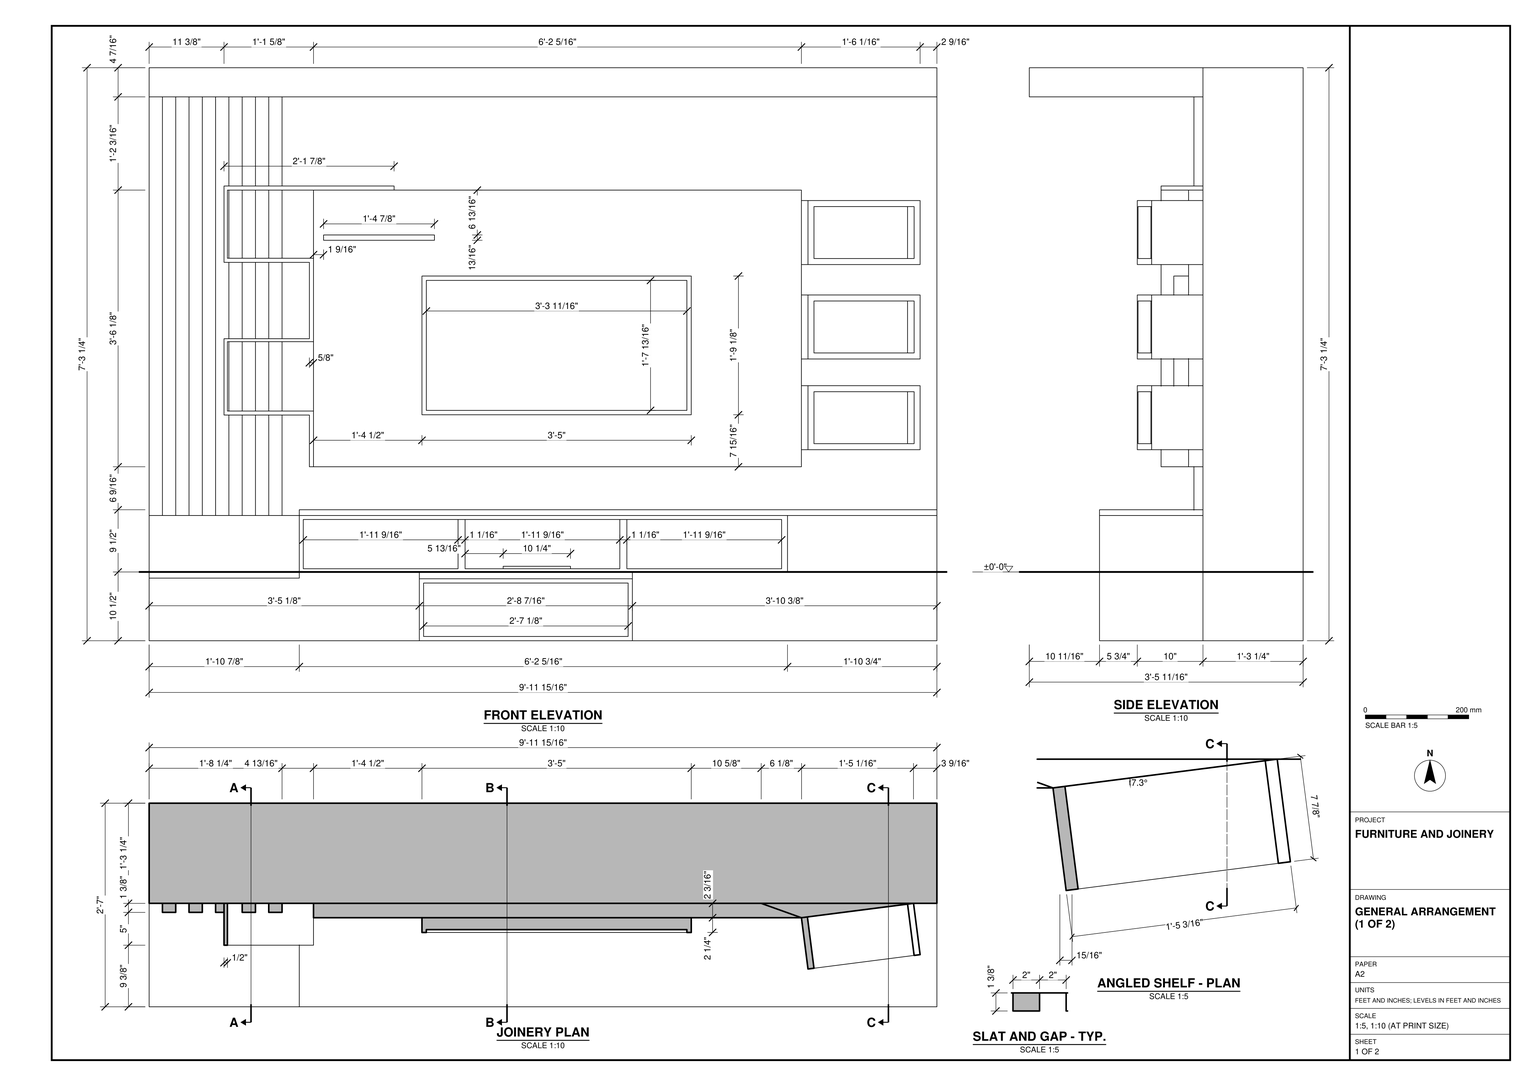
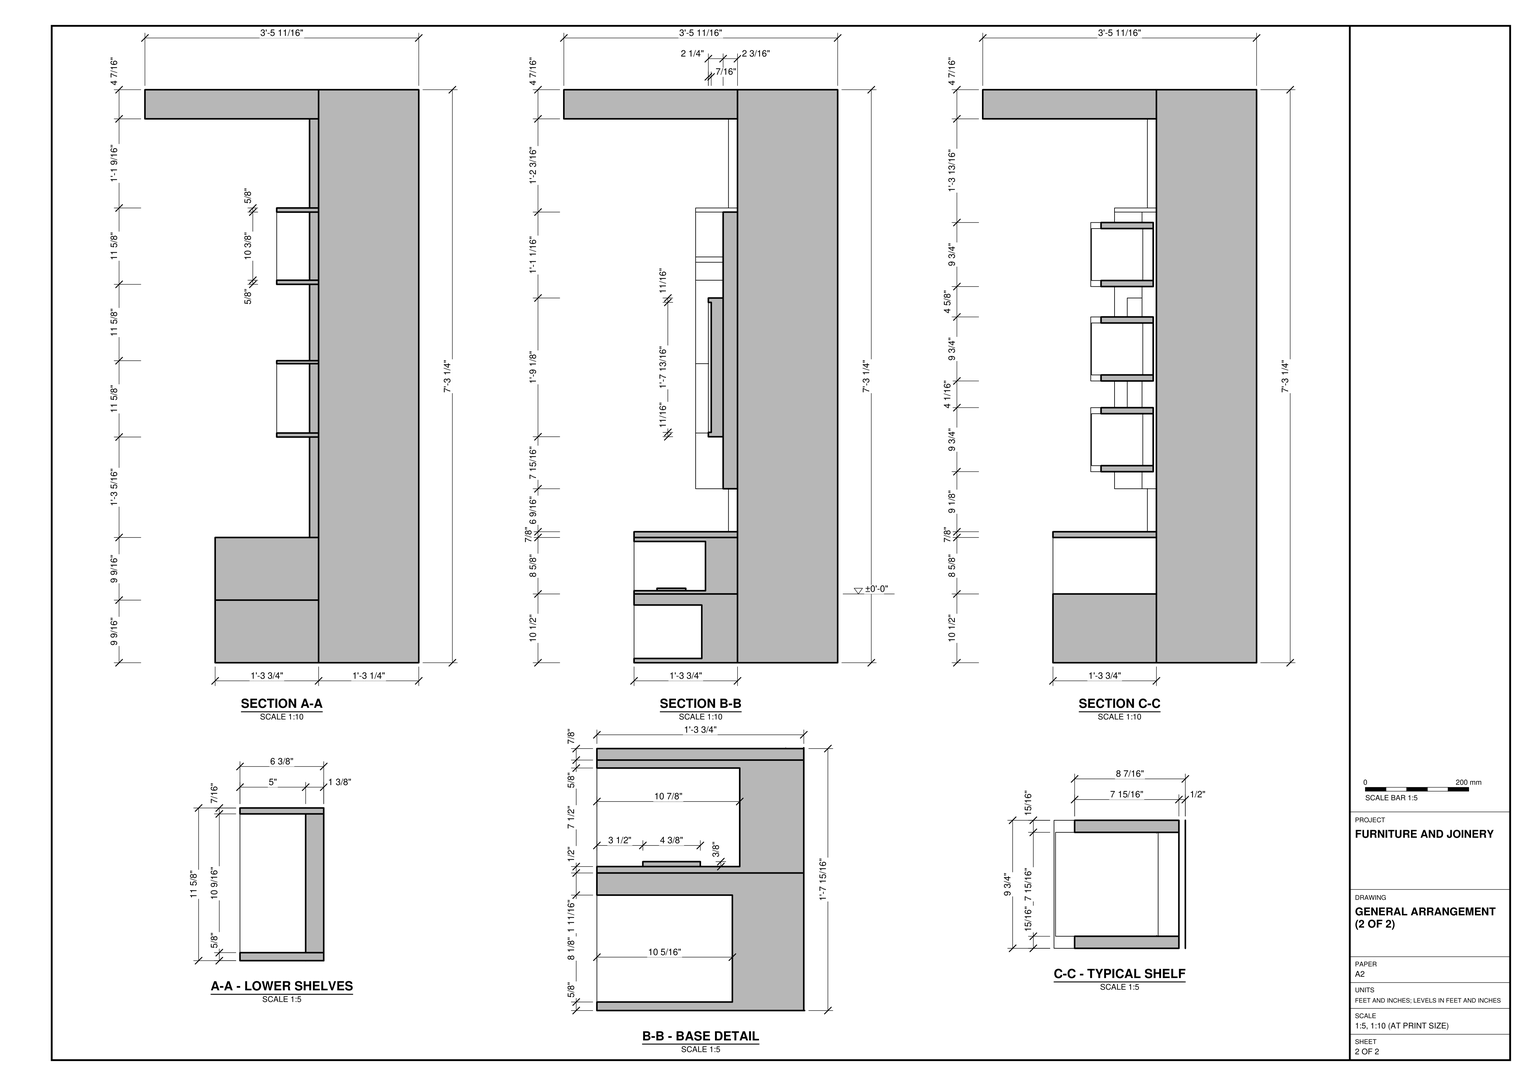
Build the media wall in SketchUp using task_files/diagram_01.pdf. Work in feet and inches. The complete unit is 9'-11 15/16" wide, 3'-5 11/16" deep and 7'-3 1/4" high. Use the ±0'-0" datum shown at the division between the two base tiers; the bottom of the unit is 10 1/2" below it.

Use the front elevation to lay out the full-height backing, the projecting top canopy and the low storage base. On the left, run the vertical slats from the base to the canopy and fit the open shelf returns in front of them. Set the broad rectangular panel forward of the backing. Include the framed display on its face and the short shelf above and to the left of the display. Stack the open box shelves at the right edge of the panel, using the angled shelf plan to orient them. In the base, form the row of three upper compartments and the wider single opening below.

Use sections A-A, B-B and C-C and their details to set board thicknesses, recess depths and projections so the joinery matches in side view as well as in elevation. Keep the backing, canopy, panel, shelving and base storage as separate groups or components, and use components for repeated parts. Any decor or loose items may be suitable library components, for example from 3D Warehouse. Save one SketchUp model as output_files/media_wall_with_display_shelving_and_base_storage.skp.

# SketchUp Ruby script. Lengths in inches.
U = 1.inch
M = Sketchup.active_model
def pt(a) = Geom::Point3d.new(a.map { |v| v * U })
def face(e, loops, mat)
  f = e.add_face(loops[0].map { |a| pt(a) })
  loops[1..].each { |l| e.add_face(l.map { |a| pt(a) }).erase! }
  f.material = f.back_material = mat if mat
  f
end
# faces: each face lists its corners as indices into pts; further lists are holes
def faces(e, pts, list, mat = nil) = list.each { |f| face(e, (f[0].is_a?(Array) ? f : [f]).map { |l| l.map { |i| pts[i] } }, mat) }
# xy, xz, yz: faces in a plane at the given z, y or x. An outline is a flat list of corners, or four numbers for a rectangle; further outlines are holes
def ring(l) = l.size == 4 ? [[l[0], l[1]], [l[2], l[1]], [l[2], l[3]], [l[0], l[3]]] : l.each_slice(2).to_a
def flat(e, list, mat, &to3) = list.each { |f| face(e, (f[0].is_a?(Array) ? f : [f]).map { |l| ring(l).map { |u, v| to3.(u, v) } }, mat) }
def xy(e, z, list, mat = nil) = flat(e, list, mat) { |x, y| [x, y, z] }
def xz(e, y, list, mat = nil) = flat(e, list, mat) { |x, z| [x, y, z] }
def yz(e, x, list, mat = nil) = flat(e, list, mat) { |y, z| [x, y, z] }
def lines(e, pts, list) = list.each { |a, b| e.add_line(pt(pts[a]), pt(pts[b])) }
# prism: a flat outline (further loops are holes) pulled along v
def prism(e, loops, v, mat = nil)
  f = face(e, loops, mat); d = Geom::Vector3d.new(v.map { |x| x * U })
  f.pushpull(f.normal.samedirection?(d) ? d.length : -d.length)
end
def box(e, o, s, mat = nil) = prism(e, [[o, [o[0] + s[0], o[1], o[2]], [o[0] + s[0], o[1] + s[1], o[2]], [o[0], o[1] + s[1], o[2]]]], [0, 0, s[2]], mat)
def at(x, y, z, deg = 0) = Geom::Transformation.translation(pt([x, y, z])) * Geom::Transformation.rotation(ORIGIN, Z_AXIS, deg.degrees)
def axes(o, x, y, z) = Geom::Transformation.new([*x, 0, *y, 0, *z, 0, *pt(o).to_a, 1])
def part(name) = M.definitions.add(name)
# library, detail: a bought-in or finely detailed component or shape, given as its bounding box
def library(name, o, s) = part(name).tap { |d| box(d.entities, o, s) }
def detail(e, o, s) = box(e.add_group.entities, o, s)
def put(e, d, t, mat = nil) = e.add_instance(d, t).tap { |i| i.material = mat if mat }
def group(e, t, mat = nil) = e.add_group.tap { |g| g.transformation = t; g.material = mat if mat }.entities
root = M.entities
M.materials.add("[0010_Snow]").color = [255, 250, 250]
M.materials.add("[Color M09]").color = [0, 0, 0]
M.materials.add("[Wood Bamboo]").color = [193, 114, 47]
M.materials.add("[Wood Bamboo]1").color = [177, 105, 43]
M.materials.add("[Wood Cherry Original]").color = [163, 92, 45]
M.materials.add("[Wood Cherry Original]1").color = [152, 86, 42]
xy(root,19.875,[[0,10.6875,119.9375,26.4375],[0,26.4375,119.9375,41.6875]])
xy(root,20.52,[[41.79,10.6875,72.92,21]],"[Wood Bamboo]")
xy(root,28.66,[[41.79,10.6875,72.92,21]],"[Wood Bamboo]")
xy(root,29.41,[[0,10.6875,22.86,26.4375]])
xy(root,30.35,[[22.86,10.6875,97.19,26.4375],[97.19,10.6875,119.9375,26.4375]])
xy(root,30.84,[[23.47,10.6875,47.03,21.5625],[[48.1,10.6875,71.66,21.5625],[53.9,14.19,64.15,18.56]],[72.73,10.6875,96.3,21.5625],[53.9,14.19,64.15,18.56]])
xy(root,31.21,[[53.9,14.19,64.15,18.56]],"[Color M09]")
xy(root,38.34,[[23.47,10.6875,47.03,21.5625],[48.1,10.6875,71.66,21.5625],[72.73,10.6875,96.3,21.5625]])
xy(root,38.94,[[0,10.6875,22.86,10.6875,22.86,26.4375,20.23,26.4375,20.23,25.0625,18.21,25.0625,18.21,26.4375,16.1875,26.4375,16.1875,25.0625,14.16,25.0625,14.16,26.4375,12.14,26.4375,12.14,25.0625,10.12,25.0625,10.12,26.4375,8.09,26.4375,8.09,25.0625,6.07,25.0625,6.07,26.4375,4.05,26.4375,4.05,25.0625,2.02,25.0625,2.02,26.4375,0,26.4375],[22.86,10.6875,97.19,26.4375],[2.02,25.0625,4.05,26.4375],[6.07,25.0625,8.09,26.4375],[10.12,25.0625,12.14,26.4375],
  [14.16,25.0625,16.1875,26.4375],[18.21,25.0625,20.23,26.4375]])
xy(root,38.94,[[97.19,10.6875,119.9375,26.4375]],"[Wood Bamboo]1")
xy(root,39.82,[[22.86,10.6875,119.9375,26.4375]],"[Wood Bamboo]1")
xy(root,46.36,[[24.4,20.0625,25.02,26.4375],[25.02,24.25,25.02,26.4375,93.18,26.4375,99.31,24.25]])
xy(root,48.96,[[100.31,16.4375,99.31,24.25,116.38,26.4375,117.38,18.625]])
xy(root,49.88,[[101.22,16.56,116.47,18.51,115.47,26.32,100.22,24.37]])
xy(root,54.24,[[11.4,20.0625,11.4,25.0625,12.14,25.0625,12.14,26.4375,14.16,26.4375,14.16,25.0625,16.1875,25.0625,16.1875,26.4375,18.21,26.4375,18.21,25.0625,20.23,25.0625,20.23,20.0625],[20.23,20.0625,24.4,26.4375],[11.4,25.0625,12.14,26.4375],[14.16,25.0625,16.1875,26.4375],[18.21,25.0625,20.23,26.4375]])
xy(root,54.85,[[11.92,20.0625,25.02,20.0625,25.02,26.4375,20.23,26.4375,20.23,25.0625,18.21,25.0625,18.21,26.4375,16.1875,26.4375,16.1875,25.0625,14.16,25.0625,14.16,26.4375,11.92,26.4375],[14.16,25.0625,16.1875,26.4375],[18.21,25.0625,20.23,26.4375]])
xy(root,57.79,[[101.22,16.56,100.22,24.37,115.47,26.32,116.47,18.51]])
xy(root,58.71,[[100.31,16.4375,117.38,18.625,116.38,26.4375,99.31,24.25]])
xy(root,62.78,[[100.31,16.4375,99.31,24.25,116.38,26.4375,117.38,18.625]])
xy(root,63.69,[[101.22,16.56,116.47,18.51,115.47,26.32,100.22,24.37]])
xy(root,65.41,[[11.92,20.0625,11.92,26.4375,14.16,26.4375,14.16,25.0625,16.1875,25.0625,16.1875,26.4375,18.21,26.4375,18.21,25.0625,20.23,25.0625,20.23,20.0625],[20.23,20.0625,25.02,26.4375],[14.16,25.0625,16.1875,26.4375],[18.21,25.0625,20.23,26.4375]])
xy(root,65.86,[[11.4,20.0625,24.4,20.0625,24.4,26.4375,20.23,26.4375,20.23,25.0625,18.21,25.0625,18.21,26.4375,16.1875,26.4375,16.1875,25.0625,14.16,25.0625,14.16,26.4375,12.14,26.4375,12.14,25.0625,11.4,25.0625],[11.4,25.0625,12.14,26.4375],[14.16,25.0625,16.1875,26.4375],[18.21,25.0625,20.23,26.4375]])
xy(root,71.61,[[101.22,16.56,100.22,24.37,115.47,26.32,116.47,18.51]])
xy(root,72.52,[[100.31,16.4375,117.38,18.625,116.38,26.4375,99.31,24.25]])
xy(root,77.15,[[100.31,16.4375,99.31,24.25,116.38,26.4375,117.38,18.625]])
xy(root,77.49,[[11.4,20.0625,11.4,25.0625,12.14,25.0625,12.14,26.4375,14.16,26.4375,14.16,25.0625,16.1875,25.0625,16.1875,26.4375,18.21,26.4375,18.21,25.0625,20.23,25.0625,20.23,20.0625],[20.23,20.0625,24.4,26.4375],[11.4,25.0625,12.14,26.4375],[14.16,25.0625,16.1875,26.4375],[18.21,25.0625,20.23,26.4375]])
xy(root,78.07,[[101.22,16.56,116.47,18.51,115.47,26.32,100.22,24.37]])
xy(root,78.11,[[11.92,20.0625,25.02,20.0625,25.02,26.4375,20.23,26.4375,20.23,25.0625,18.21,25.0625,18.21,26.4375,16.1875,26.4375,16.1875,25.0625,14.16,25.0625,14.16,26.4375,11.92,26.4375],[14.16,25.0625,16.1875,26.4375],[18.21,25.0625,20.23,26.4375]])
xy(root,80.85,[[26.56,20.0625,43.43,24.25]])
xy(root,81.66,[[26.56,20.0625,43.43,24.25]])
xy(root,85.98,[[101.22,16.56,100.22,24.37,115.47,26.32,116.47,18.51]])
xy(root,86.9,[[100.31,16.4375,117.38,18.625,116.38,26.4375,99.31,24.25]])
xy(root,88.49,[[11.92,20.0625,11.92,26.4375,14.16,26.4375,14.16,25.0625,16.1875,25.0625,16.1875,26.4375,18.21,26.4375,18.21,25.0625,20.23,25.0625,20.23,20.0625],[20.23,20.0625,25.02,26.4375],[25.02,20.0625,37.29,24.25],[25.02,24.25,37.29,26.4375],[37.29,24.25,99.31,24.25,93.18,26.4375,37.29,26.4375],
  [14.16,25.0625,16.1875,26.4375],[18.21,25.0625,20.23,26.4375]])
xy(root,89.11,[[11.4,20.0625,37.29,20.0625,37.29,26.4375,20.23,26.4375,20.23,25.0625,18.21,25.0625,18.21,26.4375,16.1875,26.4375,16.1875,25.0625,14.16,25.0625,14.16,26.4375,12.14,26.4375,12.14,25.0625,11.4,25.0625],[11.4,25.0625,12.14,26.4375],[14.16,25.0625,16.1875,26.4375],[18.21,25.0625,20.23,26.4375]])
xy(root,102.6875,[[2.02,25.0625,4.05,26.4375],[6.07,25.0625,8.09,26.4375],[10.12,25.0625,12.14,26.4375],[14.16,25.0625,16.1875,26.4375],[18.21,25.0625,20.23,26.4375]])
xy(root,102.6875,[[22.96,8.61,22.11,8.72,21.31,9.05,20.62,9.58,20.1,10.26,19.76,11.0625,19.65,11.92,19.76,12.78,20.1,13.58,20.62,14.26,21.31,14.79,22.11,15.12,22.96,15.23,23.82,15.12,24.62,14.79,25.31,14.26,25.83,13.58,26.16,12.78,26.28,11.92,26.16,11.0625,25.83,10.26,25.31,9.58,24.62,9.05,23.82,8.72],[62.28,8.61,61.42,8.72,60.62,9.05,59.93,9.58,59.41,10.26,59.08,11.0625,58.96,11.92,59.08,12.78,59.41,13.58,59.93,14.26,60.62,14.79,61.42,15.12,62.28,15.23,63.13,15.12,63.93,14.79,64.62,14.26,65.15,13.58,65.48,12.78,65.59,11.92,65.48,11.0625,65.15,10.26,64.62,9.58,63.93,9.05,63.13,8.72],[97.4,8.61,96.54,8.72,95.75,9.05,95.06,9.58,94.53,10.26,94.2,11.0625,94.09,11.92,94.2,12.78,94.53,13.58,95.06,14.26,95.75,14.79,96.54,15.12,97.4,15.23,98.26,15.12,99.06,14.79,99.74,14.26,100.27,13.58,100.6,12.78,100.71,11.92,100.6,11.0625,100.27,10.26,99.74,9.58,99.06,9.05,98.26,8.72]],"[0010_Snow]")
xy(root,102.6875,[[[0,0,0,26.4375,2.02,26.4375,2.02,25.0625,4.05,25.0625,4.05,26.4375,6.07,26.4375,6.07,25.0625,8.09,25.0625,8.09,26.4375,10.12,26.4375,10.12,25.0625,12.14,25.0625,12.14,26.4375,14.16,26.4375,14.16,25.0625,16.1875,25.0625,16.1875,26.4375,18.21,26.4375,18.21,25.0625,20.23,25.0625,20.23,26.4375,119.9375,26.4375,119.9375,0],[22.96,8.61,23.82,8.72,24.62,9.05,25.31,9.58,25.83,10.26,26.16,11.0625,26.28,11.92,26.16,12.78,25.83,13.58,25.31,14.26,24.62,14.79,23.82,15.12,22.96,15.23,22.11,15.12,21.31,14.79,20.62,14.26,20.1,13.58,19.76,12.78,19.65,11.92,19.76,11.0625,20.1,10.26,20.62,9.58,21.31,9.05,22.11,8.72],[62.28,8.61,63.13,8.72,63.93,9.05,64.62,9.58,65.15,10.26,65.48,11.0625,65.59,11.92,65.48,12.78,65.15,13.58,64.62,14.26,63.93,14.79,63.13,15.12,62.28,15.23,61.42,15.12,60.62,14.79,59.93,14.26,59.41,13.58,59.08,12.78,58.96,11.92,59.08,11.0625,59.41,10.26,59.93,9.58,60.62,9.05,61.42,8.72],[97.4,8.61,98.26,8.72,99.06,9.05,99.74,9.58,100.27,10.26,100.6,11.0625,100.71,11.92,100.6,12.78,100.27,13.58,99.74,14.26,99.06,14.79,98.26,15.12,97.4,15.23,96.54,15.12,95.75,14.79,95.06,14.26,94.53,13.58,94.2,12.78,94.09,11.92,94.2,11.0625,94.53,10.26,95.06,9.58,95.75,9.05,96.54,8.72]]],"[Wood Bamboo]")
xy(root,107.125,[[0,0,119.9375,26.4375],[0,26.4375,119.9375,41.6875]],"[Wood Bamboo]")
xz(root,0,[[0,102.6875,119.9375,107.125]],"[Wood Bamboo]")
xz(root,10.6875,[[0,19.875,41.14,19.875,41.14,30.35,22.86,30.35,22.86,29.41,0,29.41],[73.57,19.875,119.9375,30.35],[41.14,29.3125,73.57,30.35],[0,29.41,22.86,38.94],[[22.86,30.35,97.19,38.94],[23.47,30.84,23.47,38.34,96.3,38.34,96.3,30.84,72.73,30.84,72.73,38.34,71.66,38.34,71.66,30.84,48.1,30.84,48.1,38.34,47.03,38.34,47.03,30.84]]])
xz(root,10.6875,[[[41.14,19.875,73.57,29.3125],[41.79,20.52,72.92,28.66]]],"[Wood Bamboo]")
xz(root,10.6875,[[22.86,38.94,119.9375,39.82]],"[Wood Bamboo]1")
xz(root,14.19,[[53.9,30.84,64.15,31.21]],"[Color M09]")
xz(root,18.56,[[53.9,30.84,64.15,31.21]])
xz(root,20.0625,[[24.4,46.36,25.02,46.36,25.02,54.85,11.92,54.85,11.92,65.41,25.02,65.41,25.02,78.11,11.92,78.11,11.92,88.49,37.29,88.49,37.29,89.11,11.4,89.11,11.4,77.49,24.4,77.49,24.4,65.86,11.4,65.86,11.4,54.24,24.4,54.24],[26.56,80.85,43.43,81.66]])
xz(root,21,[[41.79,20.52,72.92,28.66]],"[Wood Bamboo]")
xz(root,21.5625,[[23.47,30.84,47.03,38.34],[48.1,30.84,71.66,38.34],[72.73,30.84,96.3,38.34]])
xz(root,24.25,[[41.54,54.28,82.54,75.41],[26.56,80.85,43.43,81.66]])
xz(root,24.25,[[[25.02,46.36,99.31,88.49],[41.54,54.28,82.54,75.41],[26.56,80.85,43.43,81.66]]],"[Wood Cherry Original]")
xz(root,25.0625,[[2.02,38.94,4.05,102.6875],[6.07,38.94,8.09,102.6875],[10.12,38.94,12.14,38.94,12.14,54.24,11.4,54.24,11.4,65.86,12.14,65.86,12.14,77.49,11.4,77.49,11.4,89.11,12.14,89.11,12.14,102.6875,10.12,102.6875],[14.16,38.94,16.1875,54.24],[18.21,38.94,20.23,54.24],
  [14.16,54.85,16.1875,65.41],[18.21,54.85,20.23,65.41],[14.16,65.86,16.1875,77.49],[18.21,65.86,20.23,77.49],[14.16,78.11,16.1875,88.49],
  [18.21,78.11,20.23,88.49],[14.16,89.11,16.1875,102.6875],[18.21,89.11,20.23,102.6875]],"[Wood Bamboo]")
xz(root,26.4375,[[0,19.875,0,29.41,22.86,29.41,22.86,30.35,119.9375,30.35,119.9375,19.875],[0,29.41,22.86,38.94],[22.86,30.35,97.19,38.94],[97.19,30.35,119.9375,38.94],[2.02,38.94,4.05,102.6875],
  [6.07,38.94,8.09,102.6875],[10.12,38.94,10.12,102.6875,12.14,102.6875,12.14,89.11,11.4,89.11,11.4,77.49,12.14,77.49,12.14,65.86,11.4,65.86,11.4,54.24,12.14,54.24,12.14,38.94],[14.16,38.94,16.1875,54.24],[18.21,38.94,20.23,54.24],[20.23,38.94,22.86,38.94,22.86,39.82,119.9375,39.82,119.9375,102.6875,20.23,102.6875,20.23,89.11,37.29,89.11,37.29,88.49,93.18,88.49,93.18,46.36,24.4,46.36,24.4,54.24,20.23,54.24],
  [22.86,38.94,119.9375,39.82],[24.4,46.36,24.4,54.24,20.23,54.24,20.23,54.85,25.02,54.85,25.02,46.36],[25.02,46.36,93.18,88.49],[11.4,54.24,11.4,65.86,12.14,65.86,12.14,65.41,11.92,65.41,11.92,54.85,12.14,54.85,12.14,54.24],[12.14,54.24,14.16,54.85],
  [14.16,54.24,16.1875,54.85],[16.1875,54.24,18.21,54.85],[18.21,54.24,20.23,54.85],[11.92,54.85,12.14,65.41],[14.16,54.85,16.1875,65.41],
  [18.21,54.85,20.23,65.41],[20.23,54.85,25.02,65.41],[12.14,65.41,14.16,65.86],[14.16,65.41,16.1875,65.86],[16.1875,65.41,18.21,65.86],
  [18.21,65.41,20.23,65.86],[20.23,65.41,20.23,65.86,24.4,65.86,24.4,77.49,20.23,77.49,20.23,78.11,25.02,78.11,25.02,65.41],[14.16,65.86,16.1875,77.49],[18.21,65.86,20.23,77.49],[20.23,65.86,24.4,77.49],
  [11.4,77.49,11.4,89.11,12.14,89.11,12.14,88.49,11.92,88.49,11.92,78.11,12.14,78.11,12.14,77.49],[12.14,77.49,14.16,78.11],[14.16,77.49,16.1875,78.11],[16.1875,77.49,18.21,78.11],[18.21,77.49,20.23,78.11],
  [11.92,78.11,12.14,88.49],[14.16,78.11,16.1875,88.49],[18.21,78.11,20.23,88.49],[20.23,78.11,25.02,88.49],[12.14,88.49,14.16,89.11],
  [14.16,88.49,16.1875,89.11],[16.1875,88.49,18.21,89.11],[18.21,88.49,20.23,89.11],[20.23,88.49,37.29,89.11],[14.16,89.11,16.1875,102.6875],
  [18.21,89.11,20.23,102.6875],[0,102.6875,119.9375,107.125]])
xz(root,26.4375,[[0,38.94,2.02,102.6875],[4.05,38.94,6.07,102.6875],[8.09,38.94,10.12,102.6875],[12.14,38.94,14.16,54.24],[16.1875,38.94,18.21,54.24]],"[Wood Cherry Original]")
xz(root,26.4375,[[12.14,54.85,14.16,65.41],[16.1875,54.85,18.21,65.41],[12.14,65.86,14.16,77.49],[16.1875,65.86,18.21,77.49],[12.14,78.11,14.16,88.49],
  [16.1875,78.11,18.21,88.49],[12.14,89.11,14.16,102.6875],[16.1875,89.11,18.21,102.6875]],"[Wood Cherry Original]1")
xz(root,41.6875,[[0,19.875,119.9375,107.125]],"[Wood Bamboo]")
yz(root,0,[[10.6875,19.875,26.4375,29.41],[10.6875,29.41,26.4375,38.94]])
yz(root,0,[[26.4375,19.875,41.6875,107.125],[0,102.6875,26.4375,107.125]],"[Wood Bamboo]")
yz(root,2.02,[[25.0625,38.94,26.4375,102.6875]],"[Wood Bamboo]")
yz(root,4.05,[[25.0625,38.94,26.4375,102.6875]],"[Wood Bamboo]")
yz(root,6.07,[[25.0625,38.94,26.4375,102.6875]],"[Wood Bamboo]")
yz(root,8.09,[[25.0625,38.94,26.4375,102.6875]],"[Wood Bamboo]")
yz(root,10.12,[[25.0625,38.94,26.4375,102.6875]],"[Wood Bamboo]")
yz(root,11.4,[[20.0625,54.24,25.0625,65.86],[25.0625,54.24,26.4375,65.86],[20.0625,77.49,25.0625,89.11],[25.0625,77.49,26.4375,89.11]])
yz(root,11.92,[[20.0625,54.85,26.4375,65.41],[20.0625,78.11,26.4375,88.49]])
yz(root,12.14,[[25.0625,38.94,26.4375,54.24],[25.0625,65.86,26.4375,77.49],[25.0625,89.11,26.4375,102.6875]],"[Wood Bamboo]")
yz(root,14.16,[[25.0625,38.94,26.4375,54.24],[25.0625,54.85,26.4375,65.41],[25.0625,65.86,26.4375,77.49],[25.0625,78.11,26.4375,88.49],[25.0625,89.11,26.4375,102.6875]],"[Wood Bamboo]")
yz(root,16.1875,[[25.0625,38.94,26.4375,54.24],[25.0625,54.85,26.4375,65.41],[25.0625,65.86,26.4375,77.49],[25.0625,78.11,26.4375,88.49],[25.0625,89.11,26.4375,102.6875]],"[Wood Bamboo]")
yz(root,18.21,[[25.0625,38.94,26.4375,54.24],[25.0625,54.85,26.4375,65.41],[25.0625,65.86,26.4375,77.49],[25.0625,78.11,26.4375,88.49],[25.0625,89.11,26.4375,102.6875]],"[Wood Bamboo]")
yz(root,20.23,[[25.0625,38.94,26.4375,54.24],[25.0625,54.85,26.4375,65.41],[25.0625,65.86,26.4375,77.49],[25.0625,78.11,26.4375,88.49],[25.0625,89.11,26.4375,102.6875]],"[Wood Bamboo]")
yz(root,22.86,[[10.6875,29.41,26.4375,30.35],[10.6875,30.35,26.4375,38.94]])
yz(root,22.86,[[10.6875,38.94,26.4375,39.82]],"[Wood Bamboo]1")
yz(root,23.47,[[10.6875,30.84,21.5625,38.34]])
yz(root,24.4,[[20.0625,46.36,26.4375,54.24],[20.0625,65.86,26.4375,77.49]])
yz(root,25.02,[[20.0625,46.36,24.25,54.85],[24.25,46.36,26.4375,54.85],[20.0625,65.41,24.25,78.11],[24.25,65.41,26.4375,78.11],[24.25,78.11,26.4375,88.49]])
yz(root,25.02,[[24.25,54.85,26.4375,65.41]],"[Wood Bamboo]")
yz(root,26.56,[[20.0625,80.85,24.25,81.66]])
yz(root,37.29,[[20.0625,88.49,26.4375,89.11]])
yz(root,41.79,[[10.6875,20.52,21,28.66]],"[Wood Bamboo]")
yz(root,43.43,[[20.0625,80.85,24.25,81.66]])
yz(root,47.03,[[10.6875,30.84,21.5625,38.34]])
yz(root,48.1,[[10.6875,30.84,21.5625,38.34]])
yz(root,53.9,[[14.19,30.84,18.56,31.21]],"[Color M09]")
yz(root,64.15,[[14.19,30.84,18.56,31.21]],"[Color M09]")
yz(root,71.66,[[10.6875,30.84,21.5625,38.34]])
yz(root,72.73,[[10.6875,30.84,21.5625,38.34]])
yz(root,72.92,[[10.6875,20.52,21,28.66]],"[Wood Bamboo]")
yz(root,96.3,[[10.6875,30.84,21.5625,38.34]])
yz(root,97.19,[[10.6875,30.35,26.4375,38.94]])
yz(root,119.9375,[[10.6875,19.875,26.4375,30.35]])
yz(root,119.9375,[[26.4375,19.875,41.6875,107.125],[0,102.6875,26.4375,107.125]],"[Wood Bamboo]")
yz(root,119.9375,[[10.6875,38.94,26.4375,39.82]],"[Wood Bamboo]1")
p = [[93.18,26.4375,46.36],[93.18,26.4375,88.49],[99.31,24.25,88.49],[99.31,24.25,86.9],[99.31,24.25,77.15],[99.31,24.25,72.52],
  [99.31,24.25,62.78],[99.31,24.25,58.71],[99.31,24.25,48.96],[99.31,24.25,46.36],[100.31,16.4375,48.96],[100.31,16.4375,58.71],
  [117.38,18.625,48.96],[117.38,18.625,58.71],[116.47,18.51,57.79],[116.47,18.51,49.88],[101.22,16.56,49.88],[101.22,16.56,57.79],
  [116.38,26.4375,48.96],[116.38,26.4375,58.71],[115.47,26.32,49.88],[115.47,26.32,57.79],[100.22,24.37,57.79],[100.22,24.37,49.88],
  [100.31,16.4375,62.78],[100.31,16.4375,72.52],[117.38,18.625,62.78],[117.38,18.625,72.52],[116.47,18.51,71.61],[116.47,18.51,63.69],
  [101.22,16.56,63.69],[101.22,16.56,71.61],[116.38,26.4375,62.78],[116.38,26.4375,72.52],[115.47,26.32,63.69],[115.47,26.32,71.61],
  [100.22,24.37,71.61],[100.22,24.37,63.69],[100.31,16.4375,77.15],[100.31,16.4375,86.9],[117.38,18.625,77.15],[117.38,18.625,86.9],
  [116.47,18.51,85.98],[116.47,18.51,78.07],[101.22,16.56,78.07],[101.22,16.56,85.98],[116.38,26.4375,77.15],[116.38,26.4375,86.9],
  [115.47,26.32,78.07],[115.47,26.32,85.98],[100.22,24.37,85.98],[100.22,24.37,78.07]]
faces(root,p,[[0,1,2,3,4,5,6,7,8,9],[7,8,10,11],[[10,12,13,11],[14,15,16,17]],[18,19,13,12],[[18,8,7,19],[20,21,22,23]],[23,22,17,16],[21,20,15,14],[20,21,22,23],
  [5,6,24,25],[[24,26,27,25],[28,29,30,31]],[32,33,27,26],[[32,6,5,33],[34,35,36,37]],[37,36,31,30],[35,34,29,28],[34,35,36,37],[3,4,38,39],
  [[38,40,41,39],[42,43,44,45]],[46,47,41,40],[[46,4,3,47],[48,49,50,51]],[51,50,45,44],[49,48,43,42],[48,49,50,51]])
g1 = group(root,at(41.54,22,54.28),"[Color M09]")
xy(g1,0,[[0,0,41,2.25]])
xy(g1,0.66,[[0.66,0,40.34,0.4375]])
xy(g1,20.46,[[0.66,0,40.34,0.4375]])
xy(g1,21.125,[[0,0,41,2.25]])
xz(g1,0,[[[0,0,41,21.125],[0.66,0.66,40.34,20.46]]])
xz(g1,0.4375,[[0.66,0.66,40.34,20.46]])
xz(g1,2.25,[[0,0,41,21.125]])
yz(g1,0,[[0,0,2.25,21.125]])
yz(g1,0.66,[[0,0.66,0.4375,20.46]])
yz(g1,40.34,[[0,0.66,0.4375,20.46]])
yz(g1,41,[[0,0,2.25,21.125]])
